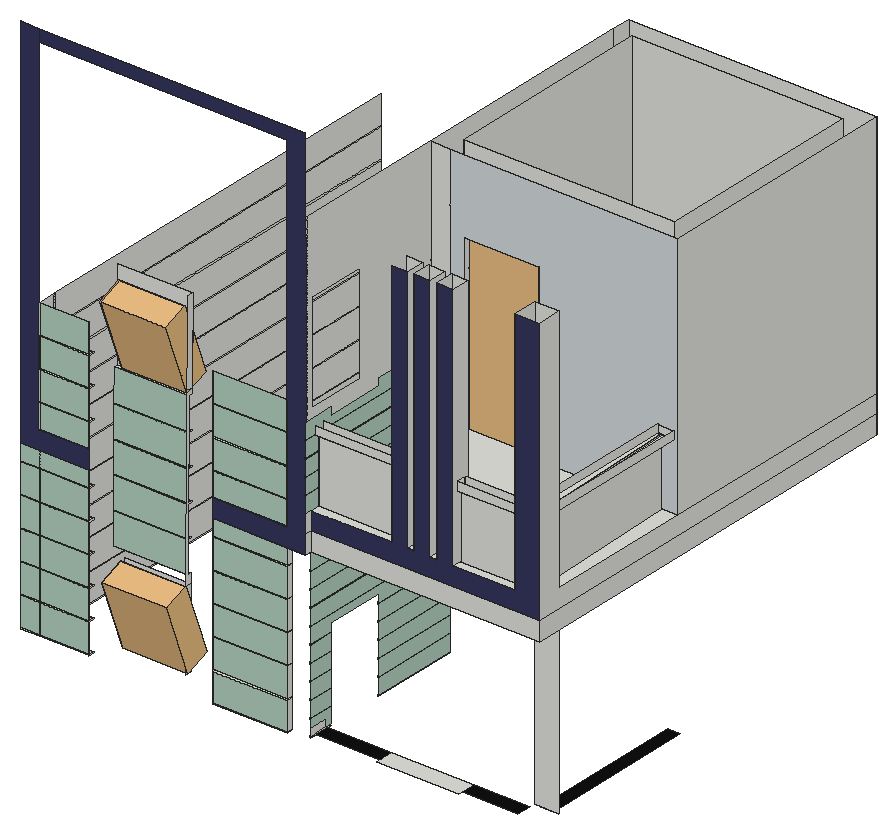
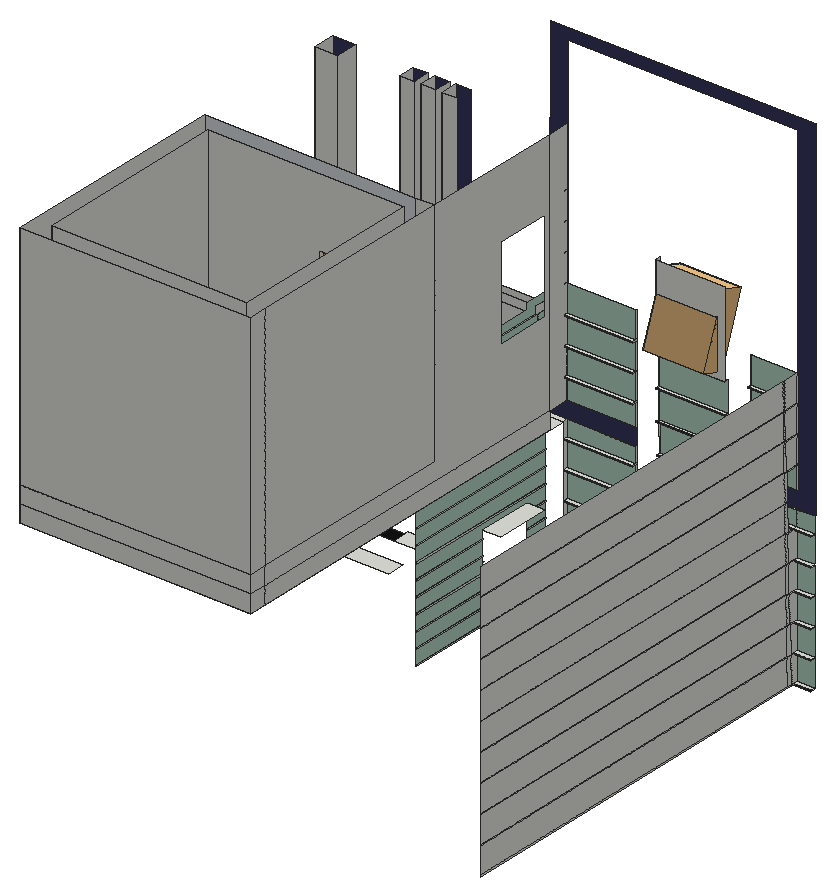
# SketchUp Ruby script. Lengths in inches.
U = 1.inch
M = Sketchup.active_model
def pt(a) = Geom::Point3d.new(a.map { |v| v * U })
def face(e, loops, mat)
  f = e.add_face(loops[0].map { |a| pt(a) })
  loops[1..].each { |l| e.add_face(l.map { |a| pt(a) }).erase! }
  f.material = f.back_material = mat if mat
  f
end
# faces: each face lists its corners as indices into pts; further lists are holes
def faces(e, pts, list, mat = nil) = list.each { |f| face(e, (f[0].is_a?(Array) ? f : [f]).map { |l| l.map { |i| pts[i] } }, mat) }
# xy, xz, yz: faces in a plane at the given z, y or x. An outline is a flat list of corners, or four numbers for a rectangle; further outlines are holes
def ring(l) = l.size == 4 ? [[l[0], l[1]], [l[2], l[1]], [l[2], l[3]], [l[0], l[3]]] : l.each_slice(2).to_a
def flat(e, list, mat, &to3) = list.each { |f| face(e, (f[0].is_a?(Array) ? f : [f]).map { |l| ring(l).map { |u, v| to3.(u, v) } }, mat) }
def xy(e, z, list, mat = nil) = flat(e, list, mat) { |x, y| [x, y, z] }
def xz(e, y, list, mat = nil) = flat(e, list, mat) { |x, z| [x, y, z] }
def yz(e, x, list, mat = nil) = flat(e, list, mat) { |y, z| [x, y, z] }
def lines(e, pts, list) = list.each { |a, b| e.add_line(pt(pts[a]), pt(pts[b])) }
# prism: a flat outline (further loops are holes) pulled along v
def prism(e, loops, v, mat = nil)
  f = face(e, loops, mat); d = Geom::Vector3d.new(v.map { |x| x * U })
  f.pushpull(f.normal.samedirection?(d) ? d.length : -d.length)
end
def box(e, o, s, mat = nil) = prism(e, [[o, [o[0] + s[0], o[1], o[2]], [o[0] + s[0], o[1] + s[1], o[2]], [o[0], o[1] + s[1], o[2]]]], [0, 0, s[2]], mat)
def at(x, y, z, deg = 0) = Geom::Transformation.translation(pt([x, y, z])) * Geom::Transformation.rotation(ORIGIN, Z_AXIS, deg.degrees)
def axes(o, x, y, z) = Geom::Transformation.new([*x, 0, *y, 0, *z, 0, *pt(o).to_a, 1])
def part(name) = M.definitions.add(name)
# library, detail: a bought-in or finely detailed component or shape, given as its bounding box
def library(name, o, s) = part(name).tap { |d| box(d.entities, o, s) }
def detail(e, o, s) = box(e.add_group.entities, o, s)
def put(e, d, t, mat = nil) = e.add_instance(d, t).tap { |i| i.material = mat if mat }
def group(e, t, mat = nil) = e.add_group.tap { |g| g.transformation = t; g.material = mat if mat }.entities
root = M.entities
M.materials.add("0235 AP 9121 dancing pink").color = [178, 209, 192]
M.materials.add("0328 AP 7205 PURPLE CHIFFON").color = [54, 55, 93]
M.materials.add("[0137_Black]").color = [17, 17, 17]
M.materials.add("[Square Glass Tile 01]").color = [212, 218, 221]
c1 = library("Group\#5",[0,0,0],[13.78,8.56,19.12])
c2 = part("Glass Door - Open Shower")
box(c2.entities,[0,0,0.95],[40,1.5,72])
c3 = library("doors",[0,-6.0625,0],[107.75,14.5625,198.25])
xy(root,177.29,[[48,70,57,72.5],[57,70,81,72.5],[141,70,177,72.5]])
xy(root,177.5,[[186,72.5,186.5,84.5],[186,113.5,186.5,156.5]])
xy(root,177.79,[[48,70,57,72.5],[57,70,81,72.5],[141,70,177,72.5]])
xy(root,178,[[186,72.5,186.5,84.5],[218.25,72.5,258.04,81.5],[186,113.5,186.5,156.5]])
xy(root,178,[[186.5,74.625,218.25,81.5],[258.04,74.75,285,81.5],[288,84.5,294.1875,161.25]],"[0137_Black]")
xy(root,185.5,[[186,72.5,186.5,84.5],[186,113.5,186.5,156.5]])
xy(root,186,[[186,72.5,186.5,84.5],[186,113.5,186.5,156.5]])
xy(root,191.23,[[141,70,177,72.5]])
xy(root,191.73,[[48,70,57,72.5],[57,70,81,72.5]])
xy(root,192.23,[[48,70,57,72.5],[57,70,81,72.5],[141,70,177,72.5]])
xy(root,193.5,[[186,72.5,186.5,84.5],[186,113.5,186.5,156.5]])
xy(root,194,[[186,72.5,186.5,84.5],[186,113.5,186.5,156.5]])
xy(root,201.5,[[186,72.5,186.5,84.5],[186,113.5,186.5,156.5]])
xy(root,202,[[186,72.5,186.5,84.5],[186,113.5,186.5,156.5]])
xy(root,206.18,[[48,70,57,72.5],[57,70,81,72.5],[141,70,177,72.5]])
xy(root,206.68,[[48,70,57,72.5],[57,70,81,72.5],[141,70,177,72.5]])
xy(root,209.5,[[186,72.5,186.5,84.5],[186,113.5,186.5,156.5]])
xy(root,210,[[186,72.5,186.5,84.5],[186,113.5,186.5,156.5]])
xy(root,217.5,[[186,72.5,186.5,84.5],[186,113.5,186.5,156.5]])
xy(root,218,[[186,72.5,186.5,84.5],[186,113.5,186.5,156.5]])
xy(root,220.63,[[48,70,57,72.5],[57,70,81,72.5],[141,70,177,72.5]])
xy(root,221.13,[[48,70,57,72.5],[57,70,81,72.5],[141,70,177,72.5]])
xy(root,222,[[177,84.5,186.5,113.5],[193.71,156.5,229.71,165.5]])
xy(root,225.5,[[186,72.5,186.5,156.5]])
xy(root,226,[[186,72.5,186.5,156.5]])
xy(root,228.63,[[92.3125,70.5,128.3125,72.5]])
xy(root,233.5,[[186,72.5,186.5,156.5]])
xy(root,234,[[186,72.5,186.5,156.5]])
xy(root,235.07,[[48,70,57,72.5],[57,70,81,72.5],[141,70,177,72.5]])
xy(root,235.57,[[48,70,57,72.5],[57,70,81,72.5],[141,70,177,72.5]])
xy(root,241.5,[[186,72.5,186.5,156.5]])
xy(root,242,[[186,72.5,186.5,156.5]])
xy(root,243.66,[[92.4,70.5,128.4,72.5]])
xy(root,244.16,[[92.4,70.5,128.4,72.5]])
xy(root,249.5,[[186,72.5,186.5,156.5]])
xy(root,249.52,[[48,70,57,72.5],[57,70,81,72.5],[141,70,177,72.5]])
xy(root,250,[[186,72.5,186.5,156.5]])
xy(root,250.02,[[48,70,57,72.5],[57,70,81,72.5],[141,70,177,72.5]])
xy(root,257.5,[[186,72.5,186.5,156.5]])
xy(root,258,[[48,69.5,57,70],[57,69.5,81,70],[141,69.5,177,70],[177,69.5,186,72.5],[186,69.5,186,156.5,297,156.5,297,84.5,285,84.5,285,72.5,186.5,72.5,186.5,69.5],
  [177,72.5,186,156.5],[285,72.5,297,84.5],[[177,156.5,297,276.5],[186,165.5,288,267.5]]])
xy(root,259.18,[[92.48,70.5,128.4,72.5],[128.4,70.5,128.48,72.5]])
xy(root,259.68,[[92.49,70.5,128.49,72.5]])
xy(root,267,[[57,69.5,81,70],[141,69.5,177,70],[177,81.5,186,81.5,186,267.5,288,267.5,288,81.5,297,81.5,297,276.5,177,276.5],[186,81.5,288,267.5]])
xy(root,274.7,[[92.57,70.5,128.57,72.5]])
xy(root,275.2,[[92.58,70.5,128.58,72.5]])
xy(root,276,[[186.5,72.5,225.39,81.5],[233.21,72.5,236.33,81.5],[244.15,72.5,247.45,81.5],[255.27,72.5,285,81.5],[186.5,81.5,285,81.5,285,84.5,297,84.5,297,156.5,229.71,156.5,229.71,165.5,193.71,165.5,193.71,156.5,186.5,156.5],
  [177,156.5,177,276.5,297,276.5,297,156.5,229.71,156.5,229.71,165.5,288,165.5,288,267.5,186,267.5,186,165.5,193.71,165.5,193.71,156.5]])
xy(root,278.42,[[57,70,81,72.5],[141,70,177,72.5]])
xy(root,278.92,[[57,70,81,72.5],[141,70,177,72.5]])
xy(root,283.5,[[186,69.5,186.5,156.5]])
xy(root,284,[[186,69.5,186.5,156.5]])
xy(root,290.23,[[92.66,70.5,128.57,72.5],[128.57,70.5,128.66,72.5]])
xy(root,290.73,[[92.66,70.5,128.66,72.5]])
xy(root,291.5,[[186,69.5,186.5,156.5]])
xy(root,292,[[186,69.5,186.5,156.5]])
xy(root,292.86,[[57,70,81,72.5],[141,70,177,72.5]])
xy(root,293.36,[[57,70,81,72.5],[141,70,177,72.5]])
xy(root,299.5,[[186,69.5,186.5,156.5]])
xy(root,300,[[186,69.5,186.5,156.5]])
xy(root,306.25,[[92.75,70.5,128.75,72.5]])
xy(root,307.31,[[57,70,81,72.5],[141,70,177,72.5]])
xy(root,307.5,[[186,69.5,186.5,156.5]])
xy(root,307.81,[[57,70,81,72.5],[141,70,177,72.5]])
xy(root,308,[[186,69.5,186.5,74.5],[185.58,74.5,186,79.5],[186,74.5,186.5,79.5],[186.5,74.5,225.39,79.5],[255.27,74.5,284.65,79.5],
  [186,79.5,186.5,156.5],[287,84.5,295,156.5]])
xz(root,69.5,[[48,258,81,258,81,267,57,267,57,441,48,441],[141,258,186.5,258,186.5,283.5,186,283.5,186,284,186.5,284,186.5,291.5,186,291.5,186,292,186.5,292,186.5,299.5,186,299.5,186,300,186.5,300,186.5,307.5,186,307.5,186,308,186.5,308,186.5,315.5,186,315.5,186,316,186.5,316,186.5,323.5,186,323.5,186,324,186.5,324,186.5,331.5,186,331.5,186,332,186.5,332,186.5,339.5,186,339.5,186,340,186.5,340,186.5,347.5,186,347.5,186,348,186.5,348,186.5,355.5,186,355.5,186,356,186.5,356,186.5,363.5,186,363.5,186,364,186.5,364,186.5,371.5,186,371.5,186,372,186.5,372,186.5,379.5,186,379.5,186,380,186.5,380,186.5,387.5,186,387.5,186,388,186.5,388,186.5,395.5,186,395.5,186,441,57,441,57,435,177,435,177,267,141,267]],"0328 AP 7205 PURPLE CHIFFON")
xz(root,70,[[48,177.79,57,191.73],[57,177.79,81,191.73],[141,177.79,177,191.23],[48,192.23,57,206.18],[57,192.23,81,206.18],
  [141,192.23,177,206.18],[48,206.68,57,220.63],[57,206.68,81,220.63],[141,206.68,177,220.63],[48,221.13,57,235.07],
  [57,221.13,81,235.07],[141,221.13,177,235.07],[48,235.57,57,249.52],[57,235.57,81,249.52],[141,235.57,177,249.52],
  [48,250.02,57,258],[57,250.02,81,258],[141,250.02,177,258],[57,267,81,278.42],[141,267,177,278.42],
  [57,278.92,81,292.86],[141,278.92,177,292.86],[57,293.36,81,307.31],[141,293.36,177,307.31],[57,307.81,81,321.76],
  [141,307.81,177,321.76]],"0235 AP 9121 dancing pink")
xz(root,70.5,[[92.3125,228.63,128.3125,228.63,128.4,243.66,92.4,243.66],[92.4,244.16,128.4,244.16,128.48,259.18,92.48,259.18],[92.49,259.68,128.49,259.68,128.57,274.7,92.57,274.7],[92.58,275.2,128.58,275.2,128.66,290.23,92.66,290.23],[92.66,290.73,128.66,290.73,128.75,306.25,92.75,306.25]],"0235 AP 9121 dancing pink")
xz(root,72.5,[[96.07,185.5,128.07,185.5,128.28,223.8125,96.28,223.8125],[186.5,258,297,267],[92.75,306.25,128.75,306.25,129,350.3125,93,350.3125]])
xz(root,72.5,[[186.5,267,297,267,297,396,285,396,285,276,255.27,276,255.27,396,247.45,396,247.45,276,244.15,276,244.15,396,236.33,396,236.33,276,233.21,276,233.21,396,225.39,396,225.39,276,186.5,276]],"0328 AP 7205 PURPLE CHIFFON")
xz(root,72.5,[[48,177.29,57,177.79],[57,177.29,81,177.79],[141,177.29,177,177.79],[141,191.23,177,192.23],[48,191.73,57,192.23],
  [57,191.73,81,192.23],[48,206.18,57,206.68],[57,206.18,81,206.68],[141,206.18,177,206.68],[48,220.63,57,221.13],
  [57,220.63,81,221.13],[141,220.63,177,221.13],[48,235.07,57,235.57],[57,235.07,81,235.57],[141,235.07,177,235.57],
  [92.4,243.66,128.4,244.16],[48,249.52,57,250.02],[57,249.52,81,250.02],[141,249.52,177,250.02],[92.48,259.18,128.48,259.18,128.49,259.68,92.49,259.68],
  [92.57,274.7,128.57,274.7,128.58,275.2,92.58,275.2],[57,278.42,81,278.92],[141,278.42,177,278.92],[92.66,290.23,128.66,290.73],[57,292.86,81,293.36],
  [141,292.86,177,293.36],[57,307.31,81,307.81],[141,307.31,177,307.81]],"[0137_Black]")
xz(root,74.5,[[185.58,308,225.39,312],[255.27,308,284.65,312]])
xz(root,79.5,[[185.58,308,225.39,312],[255.27,308,284.65,312]])
xz(root,81.5,[[225.39,276,233.21,396],[236.33,276,244.15,396],[247.45,276,255.27,396]])
xz(root,84.5,[[285,178,297,258],[[285,276,297,396],[287,308,295,312]]])
xz(root,156.5,[[177,276,186.5,276,186.5,283.5,186,283.5,186,284,186.5,284,186.5,291.5,186,291.5,186,292,186.5,292,186.5,299.5,186,299.5,186,300,186.5,300,186.5,307.5,186,307.5,186,308,186.5,308,186.5,315.5,186,315.5,186,316,186.5,316,186.5,323.5,186,323.5,186,324,186.5,324,186.5,331.5,186,331.5,186,332,186.5,332,186.5,339.5,186,339.5,186,340,186.5,340,186.5,347.5,186,347.5,186,348,186.5,348,186.5,355.5,186,355.5,186,356,186.5,356,186.5,363.5,186,363.5,186,364,186.5,364,186.5,371.5,186,371.5,186,372,186.5,372,186.5,379.5,186,379.5,186,380,186.5,380,186.5,387.5,186,387.5,186,388,186.5,388,186.5,395.5,186,395.5,186,396,177,396]])
xz(root,156.5,[[[186.5,276,193.71,276,193.71,360,229.71,360,229.71,276,297,276,297,396,186,396,186,395.5,186.5,395.5,186.5,388,186,388,186,387.5,186.5,387.5,186.5,380,186,380,186,379.5,186.5,379.5,186.5,372,186,372,186,371.5,186.5,371.5,186.5,364,186,364,186,363.5,186.5,363.5,186.5,356,186,356,186,355.5,186.5,355.5,186.5,348,186,348,186,347.5,186.5,347.5,186.5,340,186,340,186,339.5,186.5,339.5,186.5,332,186,332,186,331.5,186.5,331.5,186.5,324,186,324,186,323.5,186.5,323.5,186.5,316,186,316,186,315.5,186.5,315.5,186.5,308,186,308,186,307.5,186.5,307.5,186.5,300,186,300,186,299.5,186.5,299.5,186.5,292,186,292,186,291.5,186.5,291.5,186.5,284,186,284,186,283.5,186.5,283.5],[287,308,295,312]]],"[Square Glass Tile 01]")
xz(root,165.5,[[186,276,186,396,288,396,288,276,229.71,276,229.71,360,193.71,360,193.71,276]])
xz(root,267.5,[[186,276,288,396]])
xz(root,276.5,[[177,258,297,267],[177,267,297,276],[177,276,297,396]])
yz(root,57,[[72.5,177.29,72.5,177.79,73.88,177.79,73.87,177.29],[73.87,177.29,76.31,177.29,76.32,177.79,73.88,177.79],[76.31,177.29,76.32,177.79,276.5,177.79,276.5,177.29],[70,177.79,70,191.73,74.32,191.73,73.88,177.79],[73.88,177.79,76.32,177.79,76.62,191.73,74.32,191.73],
  [76.32,177.79,76.62,191.73,276.5,191.73,276.5,177.79],[72.5,191.73,72.5,192.23,74.34,192.23,74.32,191.73],[74.32,191.73,76.62,191.73,76.63,192.23,74.34,192.23],[76.62,191.73,76.63,192.23,276.5,192.23,276.5,191.73],[70,192.23,70,206.18,74.78,206.18,74.34,192.23],
  [74.34,192.23,76.63,192.23,76.93,206.18,74.78,206.18],[76.63,192.23,76.93,206.18,276.5,206.18,276.5,192.23],[72.5,206.18,72.5,206.68,74.8,206.68,74.78,206.18],[74.78,206.18,76.93,206.18,76.94,206.68,74.8,206.68],[76.93,206.18,76.94,206.68,276.5,206.68,276.5,206.18],
  [70,206.68,70,220.63,75.24,220.63,74.8,206.68],[74.8,206.68,76.94,206.68,77.24,220.63,75.24,220.63],[76.94,206.68,77.24,220.63,276.5,220.63,276.5,206.68],[72.5,220.63,72.5,221.13,75.25,221.13,75.24,220.63],[75.24,220.63,77.24,220.63,77.25,221.13,75.25,221.13],
  [77.24,220.63,77.25,221.13,276.5,221.13,276.5,220.63],[70,221.13,70,235.07,75.69,235.07,75.25,221.13],[75.25,221.13,77.25,221.13,77.55,235.07,75.69,235.07],[77.25,221.13,77.55,235.07,276.5,235.07,276.5,221.13],[72.5,235.07,72.5,235.57,75.71,235.57,75.69,235.07],
  [75.69,235.07,77.55,235.07,77.5625,235.57,75.71,235.57],[77.55,235.07,77.5625,235.57,276.5,235.57,276.5,235.07],[70,235.57,70,249.52,76.15,249.52,75.71,235.57],[75.71,235.57,77.5625,235.57,77.86,249.52,76.15,249.52],[77.5625,235.57,77.86,249.52,276.5,249.52,276.5,235.57],
  [72.5,249.52,72.5,250.02,76.17,250.02,76.15,249.52],[76.15,249.52,77.86,249.52,77.87,250.02,76.17,250.02],[77.86,249.52,77.87,250.02,276.5,250.02,276.5,249.52],[76.17,250.02,77.87,250.02,78.17,263.97,76.61,263.97],[77.87,250.02,78.17,263.97,276.5,263.97,276.5,250.02],
  [76.61,263.97,78.17,263.97,78.18,264.47,76.62,264.47],[78.17,263.97,78.18,264.47,276.5,264.47,276.5,263.97],[76.62,264.47,78.18,264.47,78.48,278.42,77.0625,278.42],[78.18,264.47,78.48,278.42,276.5,278.42,276.5,264.47],[69.5,267,70,278.42],
  [69.5,278.42,72.5,278.92],[72.5,278.42,72.5,278.92,77.08,278.92,77.0625,278.42],[77.0625,278.42,78.48,278.42,78.49,278.92,77.08,278.92],[78.48,278.42,78.49,278.92,276.5,278.92,276.5,278.42],[69.5,278.92,70,292.86],
  [70,278.92,70,292.86,77.52,292.86,77.08,278.92],[77.08,278.92,78.49,278.92,78.79,292.86,77.52,292.86],[78.49,278.92,78.79,292.86,276.5,292.86,276.5,278.92],[69.5,292.86,72.5,293.36],[72.5,292.86,72.5,293.36,77.53,293.36,77.52,292.86],
  [77.52,292.86,78.79,292.86,78.8,293.36,77.53,293.36],[78.79,292.86,78.8,293.36,276.5,293.36,276.5,292.86],[69.5,293.36,70,307.31],[70,293.36,70,307.31,77.97,307.31,77.53,293.36],[77.53,293.36,78.8,293.36,79.1,307.31,77.97,307.31],
  [78.8,293.36,79.1,307.31,276.5,307.31,276.5,293.36],[69.5,307.31,72.5,307.81],[72.5,307.31,72.5,307.81,77.99,307.81,77.97,307.31],[77.97,307.31,79.1,307.31,79.11,307.81,77.99,307.81],[79.1,307.31,79.11,307.81,276.5,307.81,276.5,307.31],
  [69.5,307.81,70,321.76],[70,307.81,70,321.76,78.43,321.76,77.99,307.81],[77.99,307.81,79.11,307.81,79.41,321.76,78.43,321.76],[79.11,307.81,79.41,321.76,276.5,321.76,276.5,307.81]])
yz(root,81,[[69.5,177.29,72.5,177.79],[69.5,177.79,70,191.73],[69.5,191.73,72.5,192.23],[69.5,192.23,70,206.18],[69.5,206.18,72.5,206.68],
  [69.5,206.68,70,220.63],[69.5,220.63,72.5,221.13],[69.5,221.13,70,235.07],[69.5,235.07,72.5,235.57],[69.5,235.57,70,249.52],
  [69.5,249.52,72.5,250.02],[69.5,250.02,70,258],[69.5,267,70,278.42],[69.5,278.42,72.5,278.92],[69.5,278.92,70,292.86],
  [69.5,292.86,72.5,293.36],[69.5,293.36,70,307.31],[69.5,307.31,72.5,307.81],[69.5,307.81,70,321.76]])
yz(root,141,[[69.5,177.29,72.5,177.79],[69.5,177.79,70,177.79,70,191.23,72.5,191.23,72.5,192.23,69.5,192.23],[69.5,192.23,70,206.18],[69.5,206.18,72.5,206.68],[69.5,206.68,70,220.63],
  [69.5,220.63,72.5,221.13],[69.5,221.13,70,235.07],[69.5,235.07,72.5,235.57],[69.5,235.57,70,249.52],[69.5,249.52,72.5,250.02],
  [69.5,250.02,70,258],[69.5,267,70,278.42],[69.5,278.42,72.5,278.92],[69.5,278.92,70,292.86],[69.5,292.86,72.5,293.36],
  [69.5,293.36,70,307.31],[69.5,307.31,72.5,307.81],[69.5,307.81,70,321.76]])
yz(root,177,[[70,177.79,72.5,191.23],[70,192.23,72.5,206.18],[70,206.68,72.5,220.63],[70,221.13,72.5,235.07],[70,235.57,72.5,249.52],
  [70,250.02,72.5,258],[81.5,258,267.22,267],[267.22,258,276.5,267],[69.5,267,70,278.42],[70,267,70,278.42,72.5,278.42,72.5,278.92,70,278.92,70,292.86,72.5,292.86,72.5,293.36,70,293.36,70,307.31,72.5,307.31,72.5,307.81,70,307.81,70,321.76,72.5,321.76,72.5,322.26,70,322.26,70,336.2,72.5,336.2,72.5,336.7,70,336.7,70,350.65,72.5,350.65,72.5,351.15,70,351.15,70,365.1,72.5,365.1,72.5,365.6,70,365.6,70,379.54,72.5,379.54,72.5,380.04,70,380.04,70,393.99,72.5,393.99,72.5,394.49,70,394.49,70,396,81.5,396,81.5,267],
  [[81.5,267,81.5,396,156.5,396,156.5,276,267.22,276,267.22,267],[84.5,312,113.5,360]],[267.22,267,276.5,276],[156.5,276,267.22,396],[267.22,276,276.5,396],[69.5,278.42,72.5,278.92],
  [69.5,278.92,70,292.86],[69.5,292.86,72.5,293.36],[69.5,293.36,70,307.31],[69.5,307.31,72.5,307.81],[69.5,307.81,70,321.76]])
yz(root,185.58,[[74.5,308,79.5,312]])
yz(root,186,[[72.5,177.5,84.5,178],[113.5,177.5,156.5,178],[72.5,185.5,84.5,186],[113.5,185.5,156.5,186],[72.5,193.5,84.5,194],
  [113.5,193.5,156.5,194],[72.5,201.5,84.5,202],[113.5,201.5,156.5,202],[72.5,209.5,84.5,210],[113.5,209.5,156.5,210],
  [72.5,217.5,84.5,218],[113.5,217.5,156.5,218],[72.5,225.5,156.5,226],[72.5,233.5,156.5,234],[72.5,241.5,156.5,242],
  [72.5,249.5,156.5,250],[72.5,257.5,156.5,258],[165.5,276,267.5,396],[69.5,283.5,156.5,284],[69.5,291.5,156.5,292],
  [69.5,299.5,156.5,300],[69.5,307.5,156.5,308]])
yz(root,186.5,[[74.625,177.5,81.5,178],[72.5,178,81.5,181.5],[69.5,258,72.5,267],[69.5,267,72.5,276]])
yz(root,186.5,[[81.5,178,84.5,178,84.5,185.5,72.5,185.5,72.5,181.5,81.5,181.5],[113.5,178,156.5,185.5],[72.5,186,84.5,193.5],[113.5,186,156.5,193.5],[72.5,194,84.5,201.5],
  [113.5,194,156.5,201.5],[72.5,202,84.5,209.5],[113.5,202,156.5,209.5],[72.5,210,84.5,217.5],[113.5,210,156.5,217.5],
  [72.5,218,84.5,218,84.5,222,113.5,222,113.5,218,156.5,218,156.5,225.5,72.5,225.5],[72.5,226,156.5,233.5],[72.5,234,156.5,241.5],[72.5,242,156.5,249.5],[72.5,250,156.5,257.5],
  [69.5,276,156.5,283.5],[69.5,284,156.5,291.5],[69.5,292,156.5,299.5],[69.5,300,156.5,307.5],[69.5,308,156.5,308,156.5,315.5,113.5,315.5,113.5,312,84.5,312,84.5,315.5,69.5,315.5]],"0235 AP 9121 dancing pink")
yz(root,193.71,[[156.5,276,165.5,360]])
yz(root,225.39,[[72.5,276,81.5,308],[72.5,308,74.5,312],[79.5,308,81.5,312]])
yz(root,229.71,[[156.5,276,165.5,360]])
yz(root,233.21,[[72.5,276,81.5,396]])
yz(root,236.33,[[72.5,276,81.5,396]])
yz(root,244.15,[[72.5,276,81.5,396]])
yz(root,247.45,[[72.5,276,81.5,396]])
yz(root,255.27,[[[72.5,276,81.5,396],[74.5,308,79.5,312]]])
yz(root,284.65,[[74.5,308,79.5,312]])
yz(root,285,[[72.5,276,84.5,396]])
yz(root,287,[[84.5,308,156.5,312]])
yz(root,288,[[165.5,276,267.5,396]])
yz(root,295,[[84.5,308,156.5,312]])
yz(root,297,[[72.5,258,276.5,267],[72.5,267,276.5,267,276.5,276,84.5,276,84.5,396,72.5,396],[156.5,276,276.5,396]])
p = [[128.28,72.5,223.8125],[128.07,72.5,185.5],[128.07,69.5,185.5],[128.28,69.5,223.8125],[129,72.5,350.3125],[128.75,72.5,306.25],
  [128.75,70.5,306.25],[128.66,70.5,290.73],[128.66,72.5,290.73],[128.66,72.5,290.23],[128.66,70.5,290.23],[128.58,70.5,275.2],
  [128.58,72.5,275.2],[128.57,72.5,274.7],[128.57,70.5,274.7],[128.49,70.5,259.68],[128.49,72.5,259.68],[128.48,72.5,259.18],
  [128.48,70.5,259.18],[128.4,70.5,244.16],[128.4,72.5,244.16],[128.4,72.5,243.66],[128.4,70.5,243.66],[128.3125,70.5,228.63],
  [128.3125,72.5,228.63],[129,69.5,350.3125],[285,81.5,276],[285.0625,81.5,276],[57,72.5,263.97],[57,76.61,263.97]]
faces(root,p,[[0,1,2,3],[4,5,6,7,8,9,10,11,12,13,14,15,16,17,18,19,20,21,22,23,24,0,3,25]])
lines(root,p,[[26,27],[28,29]])
put(root,c1,axes([96.47,70.79,185.42],[2.30917,0,0],[0,1.34379,0.50447],[0,-0.66905,1.7822]))
put(root,c2,axes([291.13,84.5,274.45],[-0.05205,1.79414,0],[-0.36011,-0.01045,0],[0,0,0.45988]))
put(root,c3,axes([193.71,160.82,276],[0.33411,0,0],[0,0.3128,0],[0,0,0.42371]))
put(root,c2,axes([255.27,77,275.58],[0.79375,0,0],[0,0.27223,0],[0,0,0.44444]))
put(root,c2,axes([186.5,76.94,275.58],[0.97228,0,0],[0,0.31035,0],[0,0,0.44444]))
put(root,c1,axes([96.94,69.5,307.93],[2.30917,0,0],[0,1.34379,0.50447],[0,-0.66905,1.7822]))
